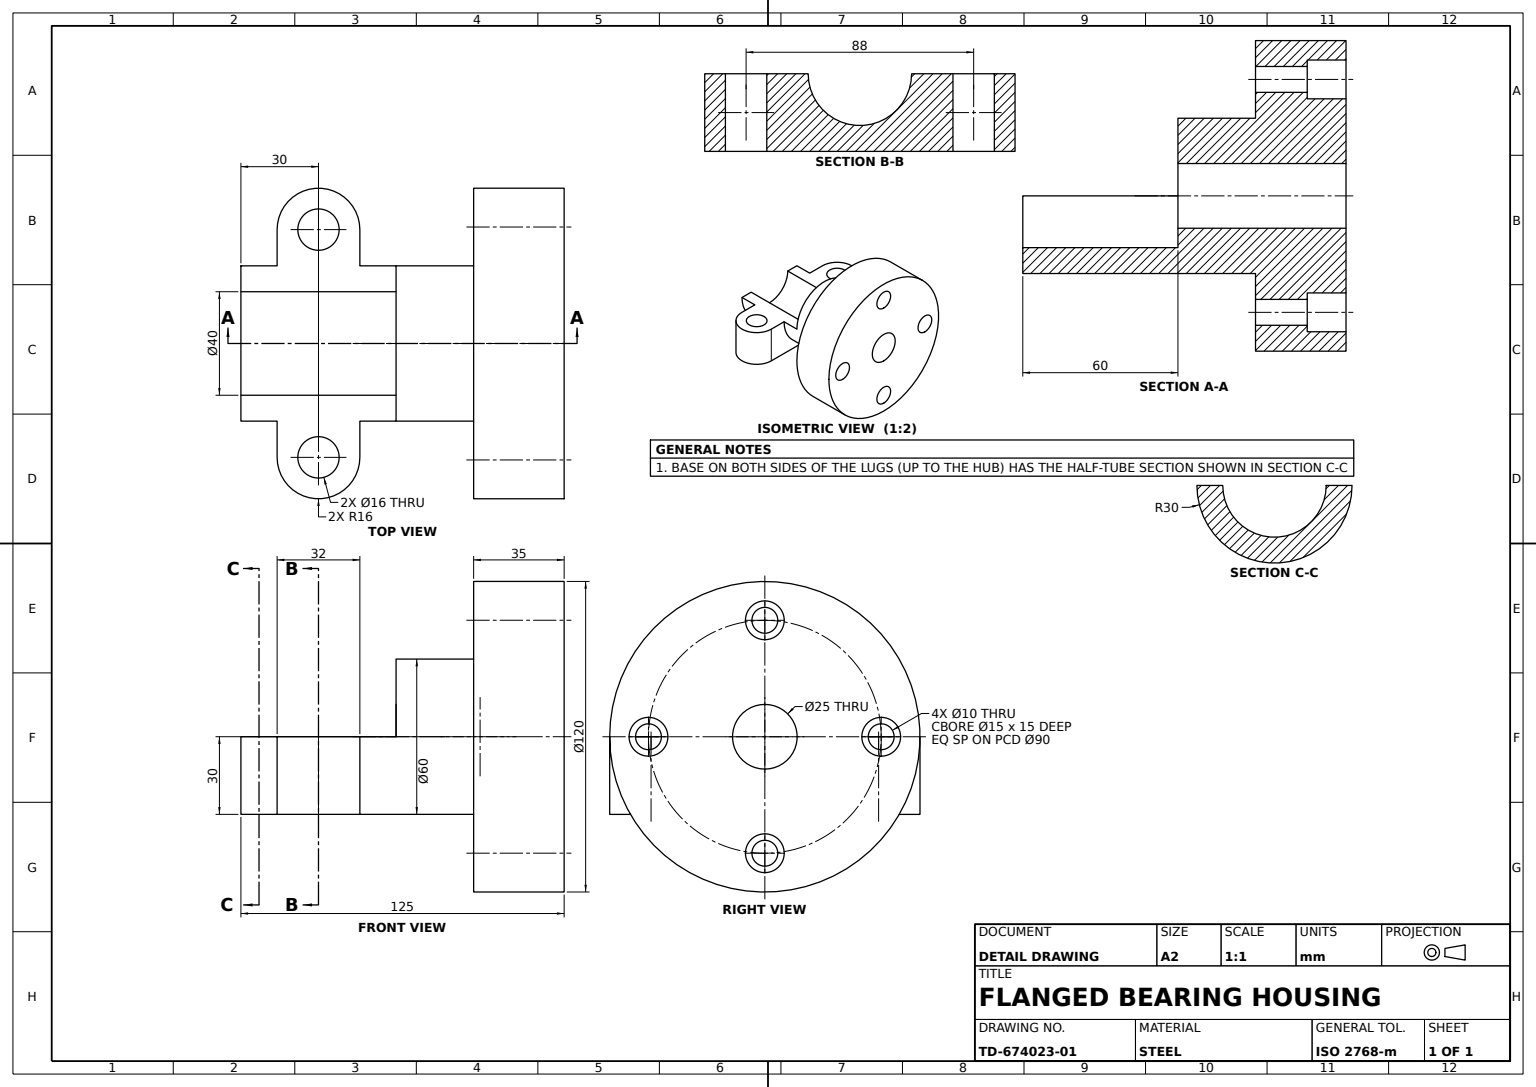
ISO-10303-21;
HEADER;
FILE_DESCRIPTION((''),'2;1');
FILE_NAME('','',(''),(''),'','','');
FILE_SCHEMA(('AUTOMOTIVE_DESIGN'));
ENDSEC;
DATA;
#1=APPLICATION_CONTEXT('');
#2=PRODUCT_CONTEXT('',#1,'mechanical');
#3=PRODUCT('','','',(#2));
#4=PRODUCT_DEFINITION_FORMATION('','',#3);
#5=PRODUCT_DEFINITION_CONTEXT('',#1,'design');
#6=PRODUCT_DEFINITION('','',#4,#5);
#7=PRODUCT_DEFINITION_SHAPE('','',#6);
#8=(LENGTH_UNIT()NAMED_UNIT(*)SI_UNIT(.MILLI.,.METRE.));
#9=(NAMED_UNIT(*)PLANE_ANGLE_UNIT()SI_UNIT($,.RADIAN.));
#10=(NAMED_UNIT(*)SI_UNIT($,.STERADIAN.)SOLID_ANGLE_UNIT());
#11=UNCERTAINTY_MEASURE_WITH_UNIT(LENGTH_MEASURE(0.005),#8,'distance_accuracy_value','');
#12=(GEOMETRIC_REPRESENTATION_CONTEXT(3)GLOBAL_UNCERTAINTY_ASSIGNED_CONTEXT((#11))GLOBAL_UNIT_ASSIGNED_CONTEXT((#8,#9,#10))REPRESENTATION_CONTEXT('',''));
#13=CARTESIAN_POINT('',(45.,-15.,-7.5));
#14=VERTEX_POINT('',#13);
#15=CARTESIAN_POINT('',(45.,-15.,0.));
#16=DIRECTION('',(0.,-1.,0.));
#17=DIRECTION('',(0.,0.,-1.));
#18=AXIS2_PLACEMENT_3D('',#15,#16,#17);
#19=CIRCLE('',#18,7.5);
#20=EDGE_CURVE('',#14,#14,#19,.F.);
#21=ORIENTED_EDGE('',*,*,#20,.F.);
#22=EDGE_LOOP('',(#21));
#23=FACE_BOUND('',#22,.T.);
#24=CARTESIAN_POINT('',(45.,0.,-7.5));
#25=VERTEX_POINT('',#24);
#26=CARTESIAN_POINT('',(45.,0.,0.));
#27=AXIS2_PLACEMENT_3D('',#26,#16,#17);
#28=CIRCLE('',#27,7.5);
#29=EDGE_CURVE('',#25,#25,#28,.T.);
#30=ORIENTED_EDGE('',*,*,#29,.F.);
#31=EDGE_LOOP('',(#30));
#32=FACE_BOUND('',#31,.T.);
#33=CYLINDRICAL_SURFACE('',#27,7.5);
#34=ADVANCED_FACE('',(#23,#32),#33,.F.);
#35=CARTESIAN_POINT('',(0.,-15.,-52.5));
#36=VERTEX_POINT('',#35);
#37=CARTESIAN_POINT('',(0.,-15.,-45.));
#38=AXIS2_PLACEMENT_3D('',#37,#16,#17);
#39=CIRCLE('',#38,7.5);
#40=EDGE_CURVE('',#36,#36,#39,.F.);
#41=ORIENTED_EDGE('',*,*,#40,.T.);
#42=EDGE_LOOP('',(#41));
#43=FACE_BOUND('',#42,.T.);
#44=CARTESIAN_POINT('',(0.,-15.,-40.));
#45=VERTEX_POINT('',#44);
#46=DIRECTION('',(0.,1.,0.));
#47=DIRECTION('',(0.,0.,1.));
#48=AXIS2_PLACEMENT_3D('',#37,#46,#47);
#49=CIRCLE('',#48,5.);
#50=EDGE_CURVE('',#45,#45,#49,.F.);
#51=ORIENTED_EDGE('',*,*,#50,.T.);
#52=EDGE_LOOP('',(#51));
#53=FACE_BOUND('',#52,.T.);
#54=PLANE('',#38);
#55=ADVANCED_FACE('',(#43,#53),#54,.F.);
#56=CARTESIAN_POINT('',(44.,-111.,-30.));
#57=VERTEX_POINT('',#56);
#58=CARTESIAN_POINT('',(0.,-111.,-30.));
#59=VERTEX_POINT('',#58);
#60=DIRECTION('',(-1.,0.,0.));
#61=VECTOR('',#60,1000.);
#62=LINE('',#56,#61);
#63=EDGE_CURVE('',#57,#59,#62,.T.);
#64=ORIENTED_EDGE('',*,*,#63,.F.);
#65=CARTESIAN_POINT('',(44.,-111.,0.));
#66=VERTEX_POINT('',#65);
#67=VECTOR('',#47,1000.);
#68=LINE('',#56,#67);
#69=EDGE_CURVE('',#66,#57,#68,.F.);
#70=ORIENTED_EDGE('',*,*,#69,.F.);
#71=CARTESIAN_POINT('',(30.,-111.,0.));
#72=VERTEX_POINT('',#71);
#73=LINE('',#65,#61);
#74=EDGE_CURVE('',#66,#72,#73,.T.);
#75=ORIENTED_EDGE('',*,*,#74,.T.);
#76=CARTESIAN_POINT('',(0.,-111.,0.));
#77=AXIS2_PLACEMENT_3D('',#76,#16,#17);
#78=CIRCLE('',#77,30.);
#79=EDGE_CURVE('',#59,#72,#78,.T.);
#80=ORIENTED_EDGE('',*,*,#79,.F.);
#81=EDGE_LOOP('',(#64,#70,#75,#80));
#82=FACE_BOUND('',#81,.T.);
#83=AXIS2_PLACEMENT_3D('',#56,#16,#17);
#84=PLANE('',#83);
#85=ADVANCED_FACE('',(#82),#84,.T.);
#86=CARTESIAN_POINT('',(0.,-15.,37.5));
#87=VERTEX_POINT('',#86);
#88=CARTESIAN_POINT('',(0.,-15.,45.));
#89=AXIS2_PLACEMENT_3D('',#88,#16,#17);
#90=CIRCLE('',#89,7.5);
#91=EDGE_CURVE('',#87,#87,#90,.F.);
#92=ORIENTED_EDGE('',*,*,#91,.F.);
#93=EDGE_LOOP('',(#92));
#94=FACE_BOUND('',#93,.T.);
#95=CARTESIAN_POINT('',(0.,0.,37.5));
#96=VERTEX_POINT('',#95);
#97=CARTESIAN_POINT('',(0.,0.,45.));
#98=AXIS2_PLACEMENT_3D('',#97,#16,#17);
#99=CIRCLE('',#98,7.5);
#100=EDGE_CURVE('',#96,#96,#99,.T.);
#101=ORIENTED_EDGE('',*,*,#100,.F.);
#102=EDGE_LOOP('',(#101));
#103=FACE_BOUND('',#102,.T.);
#104=CYLINDRICAL_SURFACE('',#98,7.5);
#105=ADVANCED_FACE('',(#94,#103),#104,.F.);
#106=CARTESIAN_POINT('',(-20.,-125.,0.));
#107=VERTEX_POINT('',#106);
#108=CARTESIAN_POINT('',(-30.,-125.,0.));
#109=VERTEX_POINT('',#108);
#110=CARTESIAN_POINT('',(-50.,-125.,0.));
#111=DIRECTION('',(1.,0.,0.));
#112=VECTOR('',#111,1000.);
#113=LINE('',#110,#112);
#114=EDGE_CURVE('',#107,#109,#113,.F.);
#115=ORIENTED_EDGE('',*,*,#114,.T.);
#116=CARTESIAN_POINT('',(30.,-125.,0.));
#117=VERTEX_POINT('',#116);
#118=CARTESIAN_POINT('',(0.,-125.,0.));
#119=AXIS2_PLACEMENT_3D('',#118,#16,#111);
#120=CIRCLE('',#119,30.);
#121=EDGE_CURVE('',#109,#117,#120,.T.);
#122=ORIENTED_EDGE('',*,*,#121,.T.);
#123=CARTESIAN_POINT('',(20.,-125.,0.));
#124=VERTEX_POINT('',#123);
#125=EDGE_CURVE('',#117,#124,#113,.F.);
#126=ORIENTED_EDGE('',*,*,#125,.T.);
#127=AXIS2_PLACEMENT_3D('',#118,#46,#47);
#128=CIRCLE('',#127,20.);
#129=EDGE_CURVE('',#124,#107,#128,.T.);
#130=ORIENTED_EDGE('',*,*,#129,.T.);
#131=EDGE_LOOP('',(#115,#122,#126,#130));
#132=FACE_BOUND('',#131,.T.);
#133=AXIS2_PLACEMENT_3D('',#118,#16,#17);
#134=PLANE('',#133);
#135=ADVANCED_FACE('',(#132),#134,.T.);
#136=ORIENTED_EDGE('',*,*,#20,.T.);
#137=EDGE_LOOP('',(#136));
#138=FACE_BOUND('',#137,.T.);
#139=CARTESIAN_POINT('',(45.,-15.,5.));
#140=VERTEX_POINT('',#139);
#141=AXIS2_PLACEMENT_3D('',#15,#46,#47);
#142=CIRCLE('',#141,5.);
#143=EDGE_CURVE('',#140,#140,#142,.F.);
#144=ORIENTED_EDGE('',*,*,#143,.T.);
#145=EDGE_LOOP('',(#144));
#146=FACE_BOUND('',#145,.T.);
#147=PLANE('',#18);
#148=ADVANCED_FACE('',(#138,#146),#147,.F.);
#149=CARTESIAN_POINT('',(0.,0.,-12.5));
#150=VERTEX_POINT('',#149);
#151=CARTESIAN_POINT('',(0.,0.,0.));
#152=AXIS2_PLACEMENT_3D('',#151,#16,#17);
#153=CIRCLE('',#152,12.5);
#154=EDGE_CURVE('',#150,#150,#153,.T.);
#155=ORIENTED_EDGE('',*,*,#154,.T.);
#156=EDGE_LOOP('',(#155));
#157=FACE_BOUND('',#156,.T.);
#158=ORIENTED_EDGE('',*,*,#100,.T.);
#159=EDGE_LOOP('',(#158));
#160=FACE_BOUND('',#159,.T.);
#161=CARTESIAN_POINT('',(-45.,0.,-7.5));
#162=VERTEX_POINT('',#161);
#163=CARTESIAN_POINT('',(-45.,0.,0.));
#164=AXIS2_PLACEMENT_3D('',#163,#16,#17);
#165=CIRCLE('',#164,7.5);
#166=EDGE_CURVE('',#162,#162,#165,.T.);
#167=ORIENTED_EDGE('',*,*,#166,.T.);
#168=EDGE_LOOP('',(#167));
#169=FACE_BOUND('',#168,.T.);
#170=ORIENTED_EDGE('',*,*,#29,.T.);
#171=EDGE_LOOP('',(#170));
#172=FACE_BOUND('',#171,.T.);
#173=CARTESIAN_POINT('',(60.,0.,0.));
#174=VERTEX_POINT('',#173);
#175=AXIS2_PLACEMENT_3D('',#151,#16,#111);
#176=CIRCLE('',#175,60.);
#177=EDGE_CURVE('',#174,#174,#176,.T.);
#178=ORIENTED_EDGE('',*,*,#177,.F.);
#179=EDGE_LOOP('',(#178));
#180=FACE_BOUND('',#179,.T.);
#181=CARTESIAN_POINT('',(0.,0.,-52.5));
#182=VERTEX_POINT('',#181);
#183=CARTESIAN_POINT('',(0.,0.,-45.));
#184=AXIS2_PLACEMENT_3D('',#183,#16,#17);
#185=CIRCLE('',#184,7.5);
#186=EDGE_CURVE('',#182,#182,#185,.T.);
#187=ORIENTED_EDGE('',*,*,#186,.T.);
#188=EDGE_LOOP('',(#187));
#189=FACE_BOUND('',#188,.T.);
#190=PLANE('',#152);
#191=ADVANCED_FACE('',(#157,#160,#169,#172,#180,#189),#190,.F.);
#192=ORIENTED_EDGE('',*,*,#186,.F.);
#193=EDGE_LOOP('',(#192));
#194=FACE_BOUND('',#193,.T.);
#195=ORIENTED_EDGE('',*,*,#40,.F.);
#196=EDGE_LOOP('',(#195));
#197=FACE_BOUND('',#196,.T.);
#198=CYLINDRICAL_SURFACE('',#184,7.5);
#199=ADVANCED_FACE('',(#194,#197),#198,.F.);
#200=ORIENTED_EDGE('',*,*,#143,.F.);
#201=EDGE_LOOP('',(#200));
#202=FACE_BOUND('',#201,.T.);
#203=CARTESIAN_POINT('',(45.,-35.,5.));
#204=VERTEX_POINT('',#203);
#205=CARTESIAN_POINT('',(45.,-35.,0.));
#206=AXIS2_PLACEMENT_3D('',#205,#46,#47);
#207=CIRCLE('',#206,5.);
#208=EDGE_CURVE('',#204,#204,#207,.T.);
#209=ORIENTED_EDGE('',*,*,#208,.F.);
#210=EDGE_LOOP('',(#209));
#211=FACE_BOUND('',#210,.T.);
#212=CYLINDRICAL_SURFACE('',#206,5.);
#213=ADVANCED_FACE('',(#202,#211),#212,.F.);
#214=CARTESIAN_POINT('',(-45.,-15.,5.));
#215=VERTEX_POINT('',#214);
#216=CARTESIAN_POINT('',(-45.,-15.,0.));
#217=AXIS2_PLACEMENT_3D('',#216,#46,#47);
#218=CIRCLE('',#217,5.);
#219=EDGE_CURVE('',#215,#215,#218,.F.);
#220=ORIENTED_EDGE('',*,*,#219,.F.);
#221=EDGE_LOOP('',(#220));
#222=FACE_BOUND('',#221,.T.);
#223=CARTESIAN_POINT('',(-45.,-35.,5.));
#224=VERTEX_POINT('',#223);
#225=CARTESIAN_POINT('',(-45.,-35.,0.));
#226=AXIS2_PLACEMENT_3D('',#225,#46,#47);
#227=CIRCLE('',#226,5.);
#228=EDGE_CURVE('',#224,#224,#227,.T.);
#229=ORIENTED_EDGE('',*,*,#228,.F.);
#230=EDGE_LOOP('',(#229));
#231=FACE_BOUND('',#230,.T.);
#232=CYLINDRICAL_SURFACE('',#226,5.);
#233=ADVANCED_FACE('',(#222,#231),#232,.F.);
#234=CARTESIAN_POINT('',(36.,-95.,-30.));
#235=VERTEX_POINT('',#234);
#236=CARTESIAN_POINT('',(44.,-95.,-30.));
#237=AXIS2_PLACEMENT_3D('',#236,#17,#60);
#238=CIRCLE('',#237,8.);
#239=EDGE_CURVE('',#235,#235,#238,.T.);
#240=ORIENTED_EDGE('',*,*,#239,.T.);
#241=EDGE_LOOP('',(#240));
#242=FACE_BOUND('',#241,.T.);
#243=CARTESIAN_POINT('',(36.,-95.,0.));
#244=VERTEX_POINT('',#243);
#245=CARTESIAN_POINT('',(44.,-95.,0.));
#246=AXIS2_PLACEMENT_3D('',#245,#17,#60);
#247=CIRCLE('',#246,8.);
#248=EDGE_CURVE('',#244,#244,#247,.T.);
#249=ORIENTED_EDGE('',*,*,#248,.F.);
#250=EDGE_LOOP('',(#249));
#251=FACE_BOUND('',#250,.T.);
#252=CYLINDRICAL_SURFACE('',#246,8.);
#253=ADVANCED_FACE('',(#242,#251),#252,.F.);
#254=CARTESIAN_POINT('',(0.,-35.,-40.));
#255=VERTEX_POINT('',#254);
#256=CARTESIAN_POINT('',(0.,-35.,-45.));
#257=AXIS2_PLACEMENT_3D('',#256,#46,#47);
#258=CIRCLE('',#257,5.);
#259=EDGE_CURVE('',#255,#255,#258,.T.);
#260=ORIENTED_EDGE('',*,*,#259,.F.);
#261=EDGE_LOOP('',(#260));
#262=FACE_BOUND('',#261,.T.);
#263=ORIENTED_EDGE('',*,*,#50,.F.);
#264=EDGE_LOOP('',(#263));
#265=FACE_BOUND('',#264,.T.);
#266=CYLINDRICAL_SURFACE('',#257,5.);
#267=ADVANCED_FACE('',(#262,#265),#266,.F.);
#268=CARTESIAN_POINT('',(-30.,-111.,0.));
#269=VERTEX_POINT('',#268);
#270=EDGE_CURVE('',#269,#59,#78,.T.);
#271=ORIENTED_EDGE('',*,*,#270,.F.);
#272=CARTESIAN_POINT('',(-44.,-111.,0.));
#273=VERTEX_POINT('',#272);
#274=EDGE_CURVE('',#269,#273,#73,.T.);
#275=ORIENTED_EDGE('',*,*,#274,.T.);
#276=CARTESIAN_POINT('',(-44.,-111.,-30.));
#277=VERTEX_POINT('',#276);
#278=LINE('',#276,#67);
#279=EDGE_CURVE('',#273,#277,#278,.F.);
#280=ORIENTED_EDGE('',*,*,#279,.T.);
#281=EDGE_CURVE('',#59,#277,#62,.T.);
#282=ORIENTED_EDGE('',*,*,#281,.F.);
#283=EDGE_LOOP('',(#271,#275,#280,#282));
#284=FACE_BOUND('',#283,.T.);
#285=ADVANCED_FACE('',(#284),#84,.T.);
#286=CARTESIAN_POINT('',(-20.,-65.,0.));
#287=VERTEX_POINT('',#286);
#288=VECTOR('',#46,1000.);
#289=LINE('',#106,#288);
#290=EDGE_CURVE('',#107,#287,#289,.T.);
#291=ORIENTED_EDGE('',*,*,#290,.F.);
#292=ORIENTED_EDGE('',*,*,#129,.F.);
#293=CARTESIAN_POINT('',(20.,-65.,0.));
#294=VERTEX_POINT('',#293);
#295=LINE('',#123,#288);
#296=EDGE_CURVE('',#294,#124,#295,.F.);
#297=ORIENTED_EDGE('',*,*,#296,.F.);
#298=CARTESIAN_POINT('',(0.,-65.,0.));
#299=AXIS2_PLACEMENT_3D('',#298,#46,#47);
#300=CIRCLE('',#299,20.);
#301=EDGE_CURVE('',#287,#294,#300,.F.);
#302=ORIENTED_EDGE('',*,*,#301,.F.);
#303=EDGE_LOOP('',(#291,#292,#297,#302));
#304=FACE_BOUND('',#303,.T.);
#305=CYLINDRICAL_SURFACE('',#127,20.);
#306=ADVANCED_FACE('',(#304),#305,.F.);
#307=CARTESIAN_POINT('',(0.,-15.,50.));
#308=VERTEX_POINT('',#307);
#309=AXIS2_PLACEMENT_3D('',#88,#46,#47);
#310=CIRCLE('',#309,5.);
#311=EDGE_CURVE('',#308,#308,#310,.F.);
#312=ORIENTED_EDGE('',*,*,#311,.F.);
#313=EDGE_LOOP('',(#312));
#314=FACE_BOUND('',#313,.T.);
#315=CARTESIAN_POINT('',(0.,-35.,50.));
#316=VERTEX_POINT('',#315);
#317=CARTESIAN_POINT('',(0.,-35.,45.));
#318=AXIS2_PLACEMENT_3D('',#317,#46,#47);
#319=CIRCLE('',#318,5.);
#320=EDGE_CURVE('',#316,#316,#319,.T.);
#321=ORIENTED_EDGE('',*,*,#320,.F.);
#322=EDGE_LOOP('',(#321));
#323=FACE_BOUND('',#322,.T.);
#324=CYLINDRICAL_SURFACE('',#318,5.);
#325=ADVANCED_FACE('',(#314,#323),#324,.F.);
#326=CARTESIAN_POINT('',(0.,-79.,-30.));
#327=VERTEX_POINT('',#326);
#328=CARTESIAN_POINT('',(-44.,-79.,-30.));
#329=VERTEX_POINT('',#328);
#330=CARTESIAN_POINT('',(44.,-79.,-30.));
#331=LINE('',#330,#61);
#332=EDGE_CURVE('',#327,#329,#331,.T.);
#333=ORIENTED_EDGE('',*,*,#332,.T.);
#334=CARTESIAN_POINT('',(-44.,-79.,0.));
#335=VERTEX_POINT('',#334);
#336=LINE('',#328,#67);
#337=EDGE_CURVE('',#329,#335,#336,.T.);
#338=ORIENTED_EDGE('',*,*,#337,.T.);
#339=CARTESIAN_POINT('',(-30.,-79.,0.));
#340=VERTEX_POINT('',#339);
#341=CARTESIAN_POINT('',(44.,-79.,0.));
#342=LINE('',#341,#61);
#343=EDGE_CURVE('',#340,#335,#342,.T.);
#344=ORIENTED_EDGE('',*,*,#343,.F.);
#345=CARTESIAN_POINT('',(0.,-79.,0.));
#346=AXIS2_PLACEMENT_3D('',#345,#46,#47);
#347=CIRCLE('',#346,30.);
#348=EDGE_CURVE('',#327,#340,#347,.T.);
#349=ORIENTED_EDGE('',*,*,#348,.F.);
#350=EDGE_LOOP('',(#333,#338,#344,#349));
#351=FACE_BOUND('',#350,.T.);
#352=AXIS2_PLACEMENT_3D('',#341,#46,#47);
#353=PLANE('',#352);
#354=ADVANCED_FACE('',(#351),#353,.T.);
#355=CARTESIAN_POINT('',(-45.,-15.,-7.5));
#356=VERTEX_POINT('',#355);
#357=AXIS2_PLACEMENT_3D('',#216,#16,#17);
#358=CIRCLE('',#357,7.5);
#359=EDGE_CURVE('',#356,#356,#358,.F.);
#360=ORIENTED_EDGE('',*,*,#359,.T.);
#361=EDGE_LOOP('',(#360));
#362=FACE_BOUND('',#361,.T.);
#363=ORIENTED_EDGE('',*,*,#219,.T.);
#364=EDGE_LOOP('',(#363));
#365=FACE_BOUND('',#364,.T.);
#366=PLANE('',#357);
#367=ADVANCED_FACE('',(#362,#365),#366,.F.);
#368=CARTESIAN_POINT('',(0.,-65.,12.5));
#369=VERTEX_POINT('',#368);
#370=CIRCLE('',#299,12.5);
#371=EDGE_CURVE('',#369,#369,#370,.T.);
#372=ORIENTED_EDGE('',*,*,#371,.F.);
#373=EDGE_LOOP('',(#372));
#374=FACE_BOUND('',#373,.T.);
#375=ORIENTED_EDGE('',*,*,#154,.F.);
#376=EDGE_LOOP('',(#375));
#377=FACE_BOUND('',#376,.T.);
#378=CYLINDRICAL_SURFACE('',#299,12.5);
#379=ADVANCED_FACE('',(#374,#377),#378,.F.);
#380=ORIENTED_EDGE('',*,*,#274,.F.);
#381=CARTESIAN_POINT('',(-30.,-65.,0.));
#382=LINE('',#381,#288);
#383=EDGE_CURVE('',#269,#109,#382,.F.);
#384=ORIENTED_EDGE('',*,*,#383,.T.);
#385=ORIENTED_EDGE('',*,*,#114,.F.);
#386=ORIENTED_EDGE('',*,*,#290,.T.);
#387=VERTEX_POINT('',#381);
#388=CARTESIAN_POINT('',(50.,-65.,0.));
#389=LINE('',#388,#61);
#390=EDGE_CURVE('',#287,#387,#389,.T.);
#391=ORIENTED_EDGE('',*,*,#390,.T.);
#392=EDGE_CURVE('',#387,#340,#382,.F.);
#393=ORIENTED_EDGE('',*,*,#392,.T.);
#394=ORIENTED_EDGE('',*,*,#343,.T.);
#395=CARTESIAN_POINT('',(-44.,-95.,0.));
#396=AXIS2_PLACEMENT_3D('',#395,#47,#60);
#397=CIRCLE('',#396,16.);
#398=EDGE_CURVE('',#335,#273,#397,.T.);
#399=ORIENTED_EDGE('',*,*,#398,.T.);
#400=EDGE_LOOP('',(#380,#384,#385,#386,#391,#393,#394,#399));
#401=FACE_BOUND('',#400,.T.);
#402=CARTESIAN_POINT('',(-52.,-95.,0.));
#403=VERTEX_POINT('',#402);
#404=AXIS2_PLACEMENT_3D('',#395,#17,#60);
#405=CIRCLE('',#404,8.);
#406=EDGE_CURVE('',#403,#403,#405,.T.);
#407=ORIENTED_EDGE('',*,*,#406,.T.);
#408=EDGE_LOOP('',(#407));
#409=FACE_BOUND('',#408,.T.);
#410=AXIS2_PLACEMENT_3D('',#151,#47,#111);
#411=PLANE('',#410);
#412=ADVANCED_FACE('',(#401,#409),#411,.T.);
#413=CARTESIAN_POINT('',(60.,-35.,0.));
#414=VERTEX_POINT('',#413);
#415=CARTESIAN_POINT('',(0.,-35.,0.));
#416=AXIS2_PLACEMENT_3D('',#415,#16,#111);
#417=CIRCLE('',#416,60.);
#418=EDGE_CURVE('',#414,#414,#417,.T.);
#419=ORIENTED_EDGE('',*,*,#418,.F.);
#420=EDGE_LOOP('',(#419));
#421=FACE_BOUND('',#420,.T.);
#422=ORIENTED_EDGE('',*,*,#177,.T.);
#423=EDGE_LOOP('',(#422));
#424=FACE_BOUND('',#423,.T.);
#425=AXIS2_PLACEMENT_3D('',#415,#46,#47);
#426=CYLINDRICAL_SURFACE('',#425,60.);
#427=ADVANCED_FACE('',(#421,#424),#426,.T.);
#428=ORIENTED_EDGE('',*,*,#248,.T.);
#429=EDGE_LOOP('',(#428));
#430=FACE_BOUND('',#429,.T.);
#431=CARTESIAN_POINT('',(30.,-65.,0.));
#432=VERTEX_POINT('',#431);
#433=EDGE_CURVE('',#432,#294,#389,.T.);
#434=ORIENTED_EDGE('',*,*,#433,.T.);
#435=ORIENTED_EDGE('',*,*,#296,.T.);
#436=ORIENTED_EDGE('',*,*,#125,.F.);
#437=LINE('',#431,#288);
#438=EDGE_CURVE('',#117,#72,#437,.T.);
#439=ORIENTED_EDGE('',*,*,#438,.T.);
#440=ORIENTED_EDGE('',*,*,#74,.F.);
#441=VERTEX_POINT('',#341);
#442=AXIS2_PLACEMENT_3D('',#245,#17,#111);
#443=CIRCLE('',#442,16.);
#444=EDGE_CURVE('',#441,#66,#443,.T.);
#445=ORIENTED_EDGE('',*,*,#444,.F.);
#446=CARTESIAN_POINT('',(30.,-79.,0.));
#447=VERTEX_POINT('',#446);
#448=EDGE_CURVE('',#441,#447,#342,.T.);
#449=ORIENTED_EDGE('',*,*,#448,.T.);
#450=EDGE_CURVE('',#447,#432,#437,.T.);
#451=ORIENTED_EDGE('',*,*,#450,.T.);
#452=EDGE_LOOP('',(#434,#435,#436,#439,#440,#445,#449,#451));
#453=FACE_BOUND('',#452,.T.);
#454=ADVANCED_FACE('',(#430,#453),#411,.T.);
#455=ORIENTED_EDGE('',*,*,#279,.F.);
#456=ORIENTED_EDGE('',*,*,#398,.F.);
#457=ORIENTED_EDGE('',*,*,#337,.F.);
#458=CARTESIAN_POINT('',(-44.,-95.,-30.));
#459=AXIS2_PLACEMENT_3D('',#458,#47,#60);
#460=CIRCLE('',#459,16.);
#461=EDGE_CURVE('',#329,#277,#460,.T.);
#462=ORIENTED_EDGE('',*,*,#461,.T.);
#463=EDGE_LOOP('',(#455,#456,#457,#462));
#464=FACE_BOUND('',#463,.T.);
#465=AXIS2_PLACEMENT_3D('',#458,#47,#111);
#466=CYLINDRICAL_SURFACE('',#465,16.);
#467=ADVANCED_FACE('',(#464),#466,.T.);
#468=ORIENTED_EDGE('',*,*,#448,.F.);
#469=VERTEX_POINT('',#330);
#470=LINE('',#330,#67);
#471=EDGE_CURVE('',#469,#441,#470,.T.);
#472=ORIENTED_EDGE('',*,*,#471,.F.);
#473=EDGE_CURVE('',#469,#327,#331,.T.);
#474=ORIENTED_EDGE('',*,*,#473,.T.);
#475=EDGE_CURVE('',#447,#327,#347,.T.);
#476=ORIENTED_EDGE('',*,*,#475,.F.);
#477=EDGE_LOOP('',(#468,#472,#474,#476));
#478=FACE_BOUND('',#477,.T.);
#479=ADVANCED_FACE('',(#478),#353,.T.);
#480=ORIENTED_EDGE('',*,*,#406,.F.);
#481=EDGE_LOOP('',(#480));
#482=FACE_BOUND('',#481,.T.);
#483=CARTESIAN_POINT('',(-52.,-95.,-30.));
#484=VERTEX_POINT('',#483);
#485=AXIS2_PLACEMENT_3D('',#458,#17,#60);
#486=CIRCLE('',#485,8.);
#487=EDGE_CURVE('',#484,#484,#486,.T.);
#488=ORIENTED_EDGE('',*,*,#487,.T.);
#489=EDGE_LOOP('',(#488));
#490=FACE_BOUND('',#489,.T.);
#491=CYLINDRICAL_SURFACE('',#404,8.);
#492=ADVANCED_FACE('',(#482,#490),#491,.F.);
#493=ORIENTED_EDGE('',*,*,#259,.T.);
#494=EDGE_LOOP('',(#493));
#495=FACE_BOUND('',#494,.T.);
#496=ORIENTED_EDGE('',*,*,#320,.T.);
#497=EDGE_LOOP('',(#496));
#498=FACE_BOUND('',#497,.T.);
#499=ORIENTED_EDGE('',*,*,#228,.T.);
#500=EDGE_LOOP('',(#499));
#501=FACE_BOUND('',#500,.T.);
#502=ORIENTED_EDGE('',*,*,#208,.T.);
#503=EDGE_LOOP('',(#502));
#504=FACE_BOUND('',#503,.T.);
#505=ORIENTED_EDGE('',*,*,#418,.T.);
#506=EDGE_LOOP('',(#505));
#507=FACE_BOUND('',#506,.T.);
#508=CARTESIAN_POINT('',(0.,-35.,-30.));
#509=VERTEX_POINT('',#508);
#510=AXIS2_PLACEMENT_3D('',#415,#16,#17);
#511=CIRCLE('',#510,30.);
#512=EDGE_CURVE('',#509,#509,#511,.F.);
#513=ORIENTED_EDGE('',*,*,#512,.T.);
#514=EDGE_LOOP('',(#513));
#515=FACE_BOUND('',#514,.T.);
#516=PLANE('',#510);
#517=ADVANCED_FACE('',(#495,#498,#501,#504,#507,#515),#516,.T.);
#518=ORIENTED_EDGE('',*,*,#311,.T.);
#519=EDGE_LOOP('',(#518));
#520=FACE_BOUND('',#519,.T.);
#521=ORIENTED_EDGE('',*,*,#91,.T.);
#522=EDGE_LOOP('',(#521));
#523=FACE_BOUND('',#522,.T.);
#524=PLANE('',#89);
#525=ADVANCED_FACE('',(#520,#523),#524,.F.);
#526=ORIENTED_EDGE('',*,*,#512,.F.);
#527=EDGE_LOOP('',(#526));
#528=FACE_BOUND('',#527,.T.);
#529=ORIENTED_EDGE('',*,*,#348,.T.);
#530=ORIENTED_EDGE('',*,*,#392,.F.);
#531=AXIS2_PLACEMENT_3D('',#298,#16,#17);
#532=CIRCLE('',#531,30.);
#533=EDGE_CURVE('',#432,#387,#532,.T.);
#534=ORIENTED_EDGE('',*,*,#533,.F.);
#535=ORIENTED_EDGE('',*,*,#450,.F.);
#536=ORIENTED_EDGE('',*,*,#475,.T.);
#537=EDGE_LOOP('',(#529,#530,#534,#535,#536));
#538=FACE_BOUND('',#537,.T.);
#539=CYLINDRICAL_SURFACE('',#299,30.);
#540=ADVANCED_FACE('',(#528,#538),#539,.T.);
#541=ORIENTED_EDGE('',*,*,#461,.F.);
#542=ORIENTED_EDGE('',*,*,#332,.F.);
#543=ORIENTED_EDGE('',*,*,#473,.F.);
#544=AXIS2_PLACEMENT_3D('',#236,#17,#111);
#545=CIRCLE('',#544,16.);
#546=EDGE_CURVE('',#469,#57,#545,.T.);
#547=ORIENTED_EDGE('',*,*,#546,.T.);
#548=ORIENTED_EDGE('',*,*,#63,.T.);
#549=ORIENTED_EDGE('',*,*,#281,.T.);
#550=EDGE_LOOP('',(#541,#542,#543,#547,#548,#549));
#551=FACE_BOUND('',#550,.T.);
#552=ORIENTED_EDGE('',*,*,#239,.F.);
#553=EDGE_LOOP('',(#552));
#554=FACE_BOUND('',#553,.T.);
#555=ORIENTED_EDGE('',*,*,#487,.F.);
#556=EDGE_LOOP('',(#555));
#557=FACE_BOUND('',#556,.T.);
#558=PLANE('',#237);
#559=ADVANCED_FACE('',(#551,#554,#557),#558,.T.);
#560=ORIENTED_EDGE('',*,*,#383,.F.);
#561=ORIENTED_EDGE('',*,*,#270,.T.);
#562=ORIENTED_EDGE('',*,*,#79,.T.);
#563=ORIENTED_EDGE('',*,*,#438,.F.);
#564=ORIENTED_EDGE('',*,*,#121,.F.);
#565=EDGE_LOOP('',(#560,#561,#562,#563,#564));
#566=FACE_BOUND('',#565,.T.);
#567=ADVANCED_FACE('',(#566),#539,.T.);
#568=ORIENTED_EDGE('',*,*,#444,.T.);
#569=ORIENTED_EDGE('',*,*,#69,.T.);
#570=ORIENTED_EDGE('',*,*,#546,.F.);
#571=ORIENTED_EDGE('',*,*,#471,.T.);
#572=EDGE_LOOP('',(#568,#569,#570,#571));
#573=FACE_BOUND('',#572,.T.);
#574=AXIS2_PLACEMENT_3D('',#236,#47,#111);
#575=CYLINDRICAL_SURFACE('',#574,16.);
#576=ADVANCED_FACE('',(#573),#575,.T.);
#577=ORIENTED_EDGE('',*,*,#371,.T.);
#578=EDGE_LOOP('',(#577));
#579=FACE_BOUND('',#578,.T.);
#580=ORIENTED_EDGE('',*,*,#301,.T.);
#581=ORIENTED_EDGE('',*,*,#433,.F.);
#582=ORIENTED_EDGE('',*,*,#533,.T.);
#583=ORIENTED_EDGE('',*,*,#390,.F.);
#584=EDGE_LOOP('',(#580,#581,#582,#583));
#585=FACE_BOUND('',#584,.T.);
#586=PLANE('',#299);
#587=ADVANCED_FACE('',(#579,#585),#586,.F.);
#588=ORIENTED_EDGE('',*,*,#359,.F.);
#589=EDGE_LOOP('',(#588));
#590=FACE_BOUND('',#589,.T.);
#591=ORIENTED_EDGE('',*,*,#166,.F.);
#592=EDGE_LOOP('',(#591));
#593=FACE_BOUND('',#592,.T.);
#594=CYLINDRICAL_SURFACE('',#164,7.5);
#595=ADVANCED_FACE('',(#590,#593),#594,.F.);
#596=CLOSED_SHELL('',(#34,#55,#85,#105,#135,#148,#191,#199,#213,#233,#253,#267,#285,#306,#325,#354,#367,#379,#412,#427,#454,#467,#479,#492,#517,#525,#540,#559,#567,#576,#587,#595));
#597=MANIFOLD_SOLID_BREP('',#596);
#598=ADVANCED_BREP_SHAPE_REPRESENTATION('',(#597),#12);
#599=SHAPE_DEFINITION_REPRESENTATION(#7,#598);
ENDSEC;
END-ISO-10303-21;
